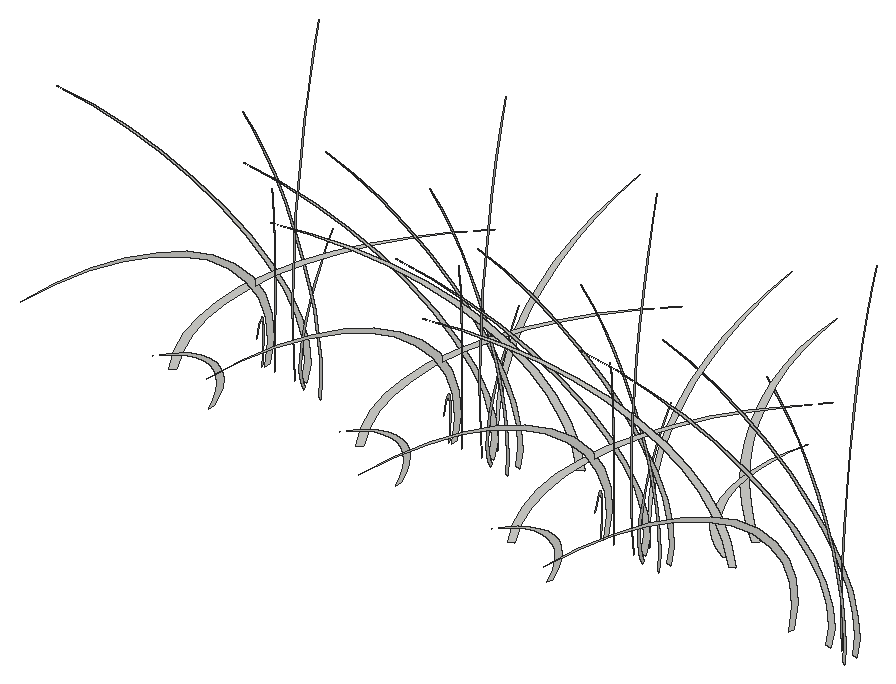
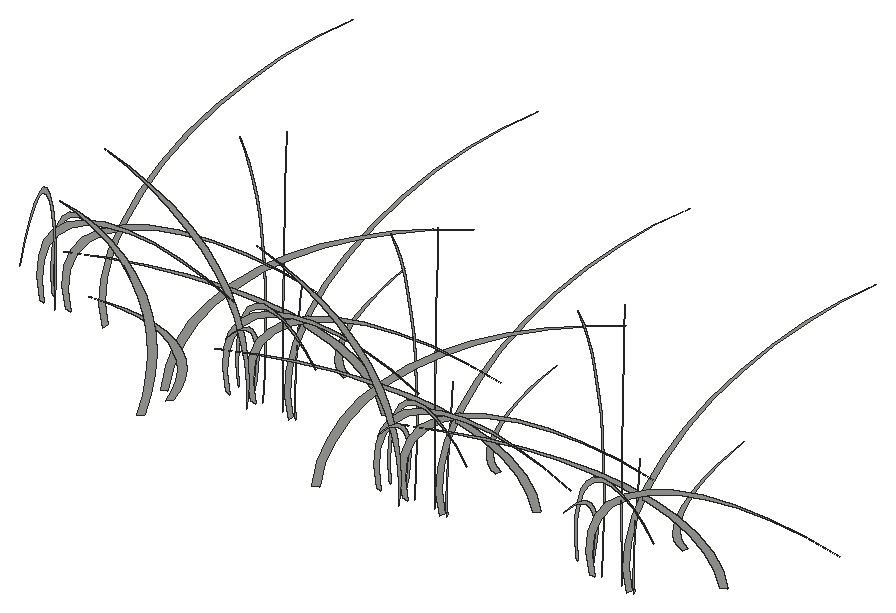
# SketchUp Ruby script. Lengths in inches.
U = 1.inch
M = Sketchup.active_model
def pt(a) = Geom::Point3d.new(a.map { |v| v * U })
def face(e, loops, mat)
  f = e.add_face(loops[0].map { |a| pt(a) })
  loops[1..].each { |l| e.add_face(l.map { |a| pt(a) }).erase! }
  f.material = f.back_material = mat if mat
  f
end
# faces: each face lists its corners as indices into pts; further lists are holes
def faces(e, pts, list, mat = nil) = list.each { |f| face(e, (f[0].is_a?(Array) ? f : [f]).map { |l| l.map { |i| pts[i] } }, mat) }
# xy, xz, yz: faces in a plane at the given z, y or x. An outline is a flat list of corners, or four numbers for a rectangle; further outlines are holes
def ring(l) = l.size == 4 ? [[l[0], l[1]], [l[2], l[1]], [l[2], l[3]], [l[0], l[3]]] : l.each_slice(2).to_a
def flat(e, list, mat, &to3) = list.each { |f| face(e, (f[0].is_a?(Array) ? f : [f]).map { |l| ring(l).map { |u, v| to3.(u, v) } }, mat) }
def xy(e, z, list, mat = nil) = flat(e, list, mat) { |x, y| [x, y, z] }
def xz(e, y, list, mat = nil) = flat(e, list, mat) { |x, z| [x, y, z] }
def yz(e, x, list, mat = nil) = flat(e, list, mat) { |y, z| [x, y, z] }
def lines(e, pts, list) = list.each { |a, b| e.add_line(pt(pts[a]), pt(pts[b])) }
# prism: a flat outline (further loops are holes) pulled along v
def prism(e, loops, v, mat = nil)
  f = face(e, loops, mat); d = Geom::Vector3d.new(v.map { |x| x * U })
  f.pushpull(f.normal.samedirection?(d) ? d.length : -d.length)
end
def box(e, o, s, mat = nil) = prism(e, [[o, [o[0] + s[0], o[1], o[2]], [o[0] + s[0], o[1] + s[1], o[2]], [o[0], o[1] + s[1], o[2]]]], [0, 0, s[2]], mat)
def at(x, y, z, deg = 0) = Geom::Transformation.translation(pt([x, y, z])) * Geom::Transformation.rotation(ORIGIN, Z_AXIS, deg.degrees)
def axes(o, x, y, z) = Geom::Transformation.new([*x, 0, *y, 0, *z, 0, *pt(o).to_a, 1])
def part(name) = M.definitions.add(name)
# library, detail: a bought-in or finely detailed component or shape, given as its bounding box
def library(name, o, s) = part(name).tap { |d| box(d.entities, o, s) }
def detail(e, o, s) = box(e.add_group.entities, o, s)
def put(e, d, t, mat = nil) = e.add_instance(d, t).tap { |i| i.material = mat if mat }
def group(e, t, mat = nil) = e.add_group.tap { |g| g.transformation = t; g.material = mat if mat }.entities
root = M.entities
g1 = group(root,at(438.46,264.24,0))
p = [[-0.1,-0.92,0],[-0.05,-0.41,0],[0,0,2.0625],[-0.02,-0.17,4.13],[-0.1,-0.9,6.16],[-0.24,-2.1875,8.1],
  [-0.44,-3.99,9.91],[-0.69,-6.27,11.52],[-0.99,-8.97,12.92],[-1.33,-12.02,14.05],[-1.69,-15.34,14.9],[-2.08,-18.86,15.45],
  [-2.48,-22.49,15.67],[-2.88,-26.13,15.5625],[-2.49,-22.56,15.58],[-2.1,-19.02,15.29],[-1.72,-15.6,14.71],[-1.37,-12.38,13.83],
  [-1.04,-9.43,12.68],[-0.75,-6.81,11.3],[-0.51,-4.6,9.7],[-0.3125,-2.84,7.9375],[-0.17,-1.5625,6.04],[-0.09,-0.81,4.05],
  [-0.07,-0.59,2.02]]
faces(g1,p,[[0,1,2,3,4,5,6,7,8,9,10,11,12,13,14,15,16,17,18,19,20,21,22,23,24]])
g2 = group(root,at(438.46,264.24,0))
p = [[-0.1,-0.92,0],[-0.05,-0.41,0],[0,0,2.0625],[-0.02,-0.17,4.13],[-0.1,-0.9,6.16],[-0.24,-2.1875,8.1],
  [-0.44,-3.99,9.91],[-0.69,-6.27,11.52],[-0.99,-8.97,12.92],[-1.33,-12.02,14.05],[-1.69,-15.34,14.9],[-2.08,-18.86,15.45],
  [-2.48,-22.49,15.67],[-2.88,-26.13,15.5625],[-2.49,-22.56,15.58],[-2.1,-19.02,15.29],[-1.72,-15.6,14.71],[-1.37,-12.38,13.83],
  [-1.04,-9.43,12.68],[-0.75,-6.81,11.3],[-0.51,-4.6,9.7],[-0.3125,-2.84,7.9375],[-0.17,-1.5625,6.04],[-0.09,-0.81,4.05],
  [-0.07,-0.59,2.02]]
faces(g2,p,[[0,1,2,3,4,5,6,7,8,9,10,11,12,13,14,15,16,17,18,19,20,21,22,23,24]])
g3 = group(root,at(419.3125,266.46,0))
p = [[-0.1,-0.92,0],[-0.05,-0.41,0],[0,0,2.0625],[-0.02,-0.17,4.13],[-0.1,-0.9,6.16],[-0.24,-2.1875,8.1],
  [-0.44,-3.99,9.91],[-0.69,-6.27,11.52],[-0.99,-8.97,12.92],[-1.33,-12.02,14.05],[-1.69,-15.34,14.9],[-2.08,-18.86,15.45],
  [-2.48,-22.49,15.67],[-2.88,-26.13,15.5625],[-2.49,-22.56,15.58],[-2.1,-19.02,15.29],[-1.72,-15.6,14.71],[-1.37,-12.38,13.83],
  [-1.04,-9.43,12.68],[-0.75,-6.81,11.3],[-0.51,-4.6,9.7],[-0.3125,-2.84,7.9375],[-0.17,-1.5625,6.04],[-0.09,-0.81,4.05],
  [-0.07,-0.59,2.02]]
faces(g3,p,[[0,1,2,3,4,5,6,7,8,9,10,11,12,13,14,15,16,17,18,19,20,21,22,23,24]])
g4 = group(root,at(419.3125,266.46,0))
p = [[-0.1,-0.92,0],[-0.05,-0.41,0],[0,0,2.0625],[-0.02,-0.17,4.13],[-0.1,-0.9,6.16],[-0.24,-2.1875,8.1],
  [-0.44,-3.99,9.91],[-0.69,-6.27,11.52],[-0.99,-8.97,12.92],[-1.33,-12.02,14.05],[-1.69,-15.34,14.9],[-2.08,-18.86,15.45],
  [-2.48,-22.49,15.67],[-2.88,-26.13,15.5625],[-2.49,-22.56,15.58],[-2.1,-19.02,15.29],[-1.72,-15.6,14.71],[-1.37,-12.38,13.83],
  [-1.04,-9.43,12.68],[-0.75,-6.81,11.3],[-0.51,-4.6,9.7],[-0.3125,-2.84,7.9375],[-0.17,-1.5625,6.04],[-0.09,-0.81,4.05],
  [-0.07,-0.59,2.02]]
faces(g4,p,[[0,1,2,3,4,5,6,7,8,9,10,11,12,13,14,15,16,17,18,19,20,21,22,23,24]])
g5 = group(root,at(420.11,259.55,0))
p = [[-0.91,-7.12,6.7],[-0.75,-5.82,6.27],[-0.6,-4.64,5.81],[-0.46,-3.6,5.31],[-0.35,-2.71,4.77],[-0.25,-1.97,4.21],
  [-0.18,-1.39,3.63],[-0.125,-0.98,3.03],[-0.09,-0.74,2.43],[-0.09,-0.67,1.8125],[-0.1,-0.77,1.2],[-0.13,-1.05,0.59],
  [-0.19,-1.49,0],[-0.12,-0.92,0],[-0.05,-0.42,0.6],[-0.01,-0.11,1.22],[0,0,1.84],[-0.01,-0.08,2.47],
  [-0.04,-0.35,3.09],[-0.1,-0.81,3.69],[-0.1875,-1.45,4.28],[-0.29,-2.27,4.84],[-0.42,-3.26,5.37],[-0.57,-4.41,5.86],
  [-0.73,-5.7,6.3]]
faces(g5,p,[[0,1,2,3,4,5,6,7,8,9,10,11,12,13,14,15,16,17,18,19,20,21,22,23,24]])
g6 = group(root,at(401.6,270.81,0))
p = [[-0.1,-0.92,0],[-0.05,-0.41,0],[0,0,2.0625],[-0.02,-0.17,4.13],[-0.1,-0.9,6.16],[-0.24,-2.1875,8.1],
  [-0.44,-3.99,9.91],[-0.69,-6.27,11.52],[-0.99,-8.97,12.92],[-1.33,-12.02,14.05],[-1.69,-15.34,14.9],[-2.08,-18.86,15.45],
  [-2.48,-22.49,15.67],[-2.88,-26.13,15.5625],[-2.49,-22.56,15.58],[-2.1,-19.02,15.29],[-1.72,-15.6,14.71],[-1.37,-12.38,13.83],
  [-1.04,-9.43,12.68],[-0.75,-6.81,11.3],[-0.51,-4.6,9.7],[-0.3125,-2.84,7.9375],[-0.17,-1.5625,6.04],[-0.09,-0.81,4.05],
  [-0.07,-0.59,2.02]]
faces(g6,p,[[0,1,2,3,4,5,6,7,8,9,10,11,12,13,14,15,16,17,18,19,20,21,22,23,24]])
g7 = group(root,at(401.6,270.81,0))
p = [[-0.1,-0.92,0],[-0.05,-0.41,0],[0,0,2.0625],[-0.02,-0.17,4.13],[-0.1,-0.9,6.16],[-0.24,-2.1875,8.1],
  [-0.44,-3.99,9.91],[-0.69,-6.27,11.52],[-0.99,-8.97,12.92],[-1.33,-12.02,14.05],[-1.69,-15.34,14.9],[-2.08,-18.86,15.45],
  [-2.48,-22.49,15.67],[-2.88,-26.13,15.5625],[-2.49,-22.56,15.58],[-2.1,-19.02,15.29],[-1.72,-15.6,14.71],[-1.37,-12.38,13.83],
  [-1.04,-9.43,12.68],[-0.75,-6.81,11.3],[-0.51,-4.6,9.7],[-0.3125,-2.84,7.9375],[-0.17,-1.5625,6.04],[-0.09,-0.81,4.05],
  [-0.07,-0.59,2.02]]
faces(g7,p,[[0,1,2,3,4,5,6,7,8,9,10,11,12,13,14,15,16,17,18,19,20,21,22,23,24]])
g8 = group(root,at(383.74,271.23,0))
p = [[-0.1,-0.92,0],[-0.05,-0.41,0],[0,0,2.0625],[-0.02,-0.17,4.13],[-0.1,-0.9,6.16],[-0.24,-2.1875,8.1],
  [-0.44,-3.99,9.91],[-0.69,-6.27,11.52],[-0.99,-8.97,12.92],[-1.33,-12.02,14.05],[-1.69,-15.34,14.9],[-2.08,-18.86,15.45],
  [-2.48,-22.49,15.67],[-2.88,-26.13,15.5625],[-2.49,-22.56,15.58],[-2.1,-19.02,15.29],[-1.72,-15.6,14.71],[-1.37,-12.38,13.83],
  [-1.04,-9.43,12.68],[-0.75,-6.81,11.3],[-0.51,-4.6,9.7],[-0.3125,-2.84,7.9375],[-0.17,-1.5625,6.04],[-0.09,-0.81,4.05],
  [-0.07,-0.59,2.02]]
faces(g8,p,[[0,1,2,3,4,5,6,7,8,9,10,11,12,13,14,15,16,17,18,19,20,21,22,23,24]])
g9 = group(root,at(383.74,271.23,0))
p = [[-0.1,-0.92,0],[-0.05,-0.41,0],[0,0,2.0625],[-0.02,-0.17,4.13],[-0.1,-0.9,6.16],[-0.24,-2.1875,8.1],
  [-0.44,-3.99,9.91],[-0.69,-6.27,11.52],[-0.99,-8.97,12.92],[-1.33,-12.02,14.05],[-1.69,-15.34,14.9],[-2.08,-18.86,15.45],
  [-2.48,-22.49,15.67],[-2.88,-26.13,15.5625],[-2.49,-22.56,15.58],[-2.1,-19.02,15.29],[-1.72,-15.6,14.71],[-1.37,-12.38,13.83],
  [-1.04,-9.43,12.68],[-0.75,-6.81,11.3],[-0.51,-4.6,9.7],[-0.3125,-2.84,7.9375],[-0.17,-1.5625,6.04],[-0.09,-0.81,4.05],
  [-0.07,-0.59,2.02]]
faces(g9,p,[[0,1,2,3,4,5,6,7,8,9,10,11,12,13,14,15,16,17,18,19,20,21,22,23,24]])
g10 = group(root,at(402.4,263.9,0))
p = [[-0.91,-7.12,6.7],[-0.75,-5.82,6.27],[-0.6,-4.64,5.81],[-0.46,-3.6,5.31],[-0.35,-2.71,4.77],[-0.25,-1.97,4.21],
  [-0.18,-1.39,3.63],[-0.125,-0.98,3.03],[-0.09,-0.74,2.43],[-0.09,-0.67,1.8125],[-0.1,-0.77,1.2],[-0.13,-1.05,0.59],
  [-0.19,-1.49,0],[-0.12,-0.92,0],[-0.05,-0.42,0.6],[-0.01,-0.11,1.22],[0,0,1.84],[-0.01,-0.08,2.47],
  [-0.04,-0.35,3.09],[-0.1,-0.81,3.69],[-0.1875,-1.45,4.28],[-0.29,-2.27,4.84],[-0.42,-3.26,5.37],[-0.57,-4.41,5.86],
  [-0.73,-5.7,6.3]]
faces(g10,p,[[0,1,2,3,4,5,6,7,8,9,10,11,12,13,14,15,16,17,18,19,20,21,22,23,24]])
g11 = group(root,at(384.54,264.32,0))
p = [[-0.91,-7.12,6.7],[-0.75,-5.82,6.27],[-0.6,-4.64,5.81],[-0.46,-3.6,5.31],[-0.35,-2.71,4.77],[-0.25,-1.97,4.21],
  [-0.18,-1.39,3.63],[-0.125,-0.98,3.03],[-0.09,-0.74,2.43],[-0.09,-0.67,1.8125],[-0.1,-0.77,1.2],[-0.13,-1.05,0.59],
  [-0.19,-1.49,0],[-0.12,-0.92,0],[-0.05,-0.42,0.6],[-0.01,-0.11,1.22],[0,0,1.84],[-0.01,-0.08,2.47],
  [-0.04,-0.35,3.09],[-0.1,-0.81,3.69],[-0.1875,-1.45,4.28],[-0.29,-2.27,4.84],[-0.42,-3.26,5.37],[-0.57,-4.41,5.86],
  [-0.73,-5.7,6.3]]
faces(g11,p,[[0,1,2,3,4,5,6,7,8,9,10,11,12,13,14,15,16,17,18,19,20,21,22,23,24]])
g12 = group(root,at(419.68,266.18,0))
p = [[0.57,-0.76,0],[0.25,-0.34,1.67],[0.0625,-0.09,3.36],[0,0,5.0625],[0.0625,-0.08,6.76],[0.25,-0.33,8.45],
  [0.5625,-0.75,10.12],[1,-1.34,11.77],[1.56,-2.08,13.4],[2.23,-2.99,14.98],[3.03,-4.05,16.53],[3.93,-5.26,18.02],
  [4.95,-6.62,19.46],[3.99,-5.34,18],[3.14,-4.2,16.49],[2.39,-3.19,14.9375],[1.74,-2.33,13.35],[1.2,-1.61,11.73],
  [0.77,-1.03,10.08],[0.46,-0.61,8.42],[0.25,-0.34,6.74],[0.16,-0.21,5.05],[0.18,-0.24,3.36],[0.32,-0.43,1.68]]
faces(g12,p,[[0,1,2,3,4,5,6,7,8,9,10,11,12,13,14,15,16,17,18,19,20,21,22,23]])
g13 = group(root,at(418.05,266.83,0))
p = [[5.52,-7.72,6.7],[4.47,-6.25,6.27],[3.52,-4.92,5.81],[2.68,-3.75,5.31],[1.96,-2.74,4.77],[1.37,-1.91,4.21],
  [0.9,-1.26,3.63],[0.57,-0.79,3.03],[0.37,-0.52,2.43],[0.31,-0.44,1.8125],[0.4,-0.56,1.2],[0.62,-0.87,0.59],
  [0.98,-1.37,0],[0.74,-1.03,0],[0.33,-0.46,0.59],[0.07,-0.1,1.19],[-0.04,0.05,1.81],[0.01,-0.02,2.43],
  [0.21,-0.3,3.04],[0.5625,-0.79,3.65],[1.0625,-1.49,4.23],[1.7,-2.38,4.8],[2.48,-3.47,5.33],[3.38,-4.73,5.83],
  [4.4,-6.15,6.29]]
faces(g13,p,[[0,1,2,3,4,5,6,7,8,9,10,11,12,13,14,15,16,17,18,19,20,21,22,23,24]])
g14 = group(root,at(429.37,268.4,0))
p = [[-19.18,-7.98,16.73],[-22.08,-9.1875,17.17],[-19.27,-8.02,16.64],[-16.57,-6.9,15.9],[-13.98,-5.82,14.96],[-11.56,-4.8125,13.84],
  [-9.32,-3.88,12.54],[-7.28,-3.03,11.08],[-5.47,-2.28,9.48],[-3.92,-1.63,7.76],[-2.63,-1.09,5.92],[-1.625,-0.68,4.01],
  [-0.91,-0.38,2.02],[-0.5,-0.21,0],[0,0,0],[-0.34,-0.14,2.07],[-1.01,-0.42,4.1],[-1.99,-0.83,6.07],
  [-3.29,-1.37,7.94],[-4.88,-2.03,9.7],[-6.74,-2.81,11.33],[-8.85,-3.68,12.79],[-11.18,-4.65,14.08],[-13.7,-5.7,15.17],
  [-16.375,-6.82,16.0625]]
faces(g14,p,[[0,1,2,3,4,5,6,7,8,9,10,11,12,13,14,15,16,17,18,19,20,21,22,23,24]])
g15 = group(root,at(442.7,263.3,0))
p = [[-0.98,0.17,0],[-0.43,0.08,0],[0,0,1.75],[-0.18,0.03,3.51],[-0.96,0.17,5.24],[-2.32,0.41,6.89],
  [-4.24,0.76,8.42],[-6.67,1.1875,9.8],[-9.54,1.7,10.98],[-12.78,2.28,11.95],[-16.32,2.91,12.67],[-20.06,3.57,13.13],
  [-23.91,4.26,13.32],[-27.78,4.95,13.23],[-23.98,4.27,13.25],[-20.22,3.6,13],[-16.59,2.96,12.5],[-13.16,2.34,11.75],
  [-10.02,1.79,10.78],[-7.25,1.29,9.6],[-4.89,0.87,8.25],[-3.02,0.54,6.75],[-1.66,0.3,5.13],[-0.86,0.15,3.44],
  [-0.63,0.11,1.72]]
faces(g15,p,[[0,1,2,3,4,5,6,7,8,9,10,11,12,13,14,15,16,17,18,19,20,21,22,23,24]])
g16 = group(root,at(442.7,263.3,0))
p = [[-0.98,0.17,0],[-0.43,0.08,0],[0,0,1.75],[-0.18,0.03,3.51],[-0.96,0.17,5.24],[-2.32,0.41,6.89],
  [-4.24,0.76,8.42],[-6.67,1.1875,9.8],[-9.54,1.7,10.98],[-12.78,2.28,11.95],[-16.32,2.91,12.67],[-20.06,3.57,13.13],
  [-23.91,4.26,13.32],[-27.78,4.95,13.23],[-23.98,4.27,13.25],[-20.22,3.6,13],[-16.59,2.96,12.5],[-13.16,2.34,11.75],
  [-10.02,1.79,10.78],[-7.25,1.29,9.6],[-4.89,0.87,8.25],[-3.02,0.54,6.75],[-1.66,0.3,5.13],[-0.86,0.15,3.44],
  [-0.63,0.11,1.72]]
faces(g16,p,[[0,1,2,3,4,5,6,7,8,9,10,11,12,13,14,15,16,17,18,19,20,21,22,23,24]])
g17 = group(root,at(401.97,270.53,0))
p = [[0.57,-0.76,0],[0.25,-0.34,1.67],[0.0625,-0.09,3.36],[0,0,5.0625],[0.0625,-0.08,6.76],[0.25,-0.33,8.45],
  [0.5625,-0.75,10.12],[1,-1.34,11.77],[1.56,-2.08,13.4],[2.23,-2.99,14.98],[3.03,-4.05,16.53],[3.93,-5.26,18.02],
  [4.95,-6.62,19.46],[3.99,-5.34,18],[3.14,-4.2,16.49],[2.39,-3.19,14.9375],[1.74,-2.33,13.35],[1.2,-1.61,11.73],
  [0.77,-1.03,10.08],[0.46,-0.61,8.42],[0.25,-0.34,6.74],[0.16,-0.21,5.05],[0.18,-0.24,3.36],[0.32,-0.43,1.68]]
faces(g17,p,[[0,1,2,3,4,5,6,7,8,9,10,11,12,13,14,15,16,17,18,19,20,21,22,23]])
g18 = group(root,at(400.35,271.18,0))
p = [[5.52,-7.72,6.7],[4.47,-6.25,6.27],[3.52,-4.92,5.81],[2.68,-3.75,5.31],[1.96,-2.74,4.77],[1.37,-1.91,4.21],
  [0.9,-1.26,3.63],[0.57,-0.79,3.03],[0.37,-0.52,2.43],[0.31,-0.44,1.8125],[0.4,-0.56,1.2],[0.62,-0.87,0.59],
  [0.98,-1.37,0],[0.74,-1.03,0],[0.33,-0.46,0.59],[0.07,-0.1,1.19],[-0.04,0.05,1.81],[0.01,-0.02,2.43],
  [0.21,-0.3,3.04],[0.5625,-0.79,3.65],[1.0625,-1.49,4.23],[1.7,-2.38,4.8],[2.48,-3.47,5.33],[3.38,-4.73,5.83],
  [4.4,-6.15,6.29]]
faces(g18,p,[[0,1,2,3,4,5,6,7,8,9,10,11,12,13,14,15,16,17,18,19,20,21,22,23,24]])
g19 = group(root,at(384.11,270.95,0))
p = [[0.57,-0.76,0],[0.25,-0.34,1.67],[0.0625,-0.09,3.36],[0,0,5.0625],[0.0625,-0.08,6.76],[0.25,-0.33,8.45],
  [0.5625,-0.75,10.12],[1,-1.34,11.77],[1.56,-2.08,13.4],[2.23,-2.99,14.98],[3.03,-4.05,16.53],[3.93,-5.26,18.02],
  [4.95,-6.62,19.46],[3.99,-5.34,18],[3.14,-4.2,16.49],[2.39,-3.19,14.9375],[1.74,-2.33,13.35],[1.2,-1.61,11.73],
  [0.77,-1.03,10.08],[0.46,-0.61,8.42],[0.25,-0.34,6.74],[0.16,-0.21,5.05],[0.18,-0.24,3.36],[0.32,-0.43,1.68]]
faces(g19,p,[[0,1,2,3,4,5,6,7,8,9,10,11,12,13,14,15,16,17,18,19,20,21,22,23]])
g20 = group(root,at(413.92,260.93,0))
p = [[17.17,11.7,12.375],[19.76,13.47,12.7],[17.25,11.76,12.31],[14.83,10.11,11.76],[12.52,8.53,11.07],[10.35,7.05,10.23],
  [8.34,5.68,9.27],[6.52,4.44,8.2],[4.9,3.34,7.01],[3.51,2.39,5.74],[2.35,1.6,4.38],[1.45,0.99,2.96],
  [0.82,0.56,1.5],[0.45,0.3,0],[0,0,0],[0.3,0.21,1.53],[0.9,0.61,3.03],[1.78,1.22,4.49],
  [2.95,2.01,5.875],[4.37,2.98,7.18],[6.03,4.11,8.375],[7.92,5.4,9.46],[10,6.82,10.41],[12.26,8.36,11.22],
  [14.66,9.99,11.88]]
faces(g20,p,[[0,1,2,3,4,5,6,7,8,9,10,11,12,13,14,15,16,17,18,19,20,21,22,23,24]])
g21 = group(root,at(382.48,271.6,0))
p = [[5.52,-7.72,6.7],[4.47,-6.25,6.27],[3.52,-4.92,5.81],[2.68,-3.75,5.31],[1.96,-2.74,4.77],[1.37,-1.91,4.21],
  [0.9,-1.26,3.63],[0.57,-0.79,3.03],[0.37,-0.52,2.43],[0.31,-0.44,1.8125],[0.4,-0.56,1.2],[0.62,-0.87,0.59],
  [0.98,-1.37,0],[0.74,-1.03,0],[0.33,-0.46,0.59],[0.07,-0.1,1.19],[-0.04,0.05,1.81],[0.01,-0.02,2.43],
  [0.21,-0.3,3.04],[0.5625,-0.79,3.65],[1.0625,-1.49,4.23],[1.7,-2.38,4.8],[2.48,-3.47,5.33],[3.38,-4.73,5.83],
  [4.4,-6.15,6.29]]
faces(g21,p,[[0,1,2,3,4,5,6,7,8,9,10,11,12,13,14,15,16,17,18,19,20,21,22,23,24]])
g22 = group(root,at(424.125,263.46,0))
p = [[-3.85,8.68,9.0625],[-3.11,7.03,8.49],[-2.45,5.54,7.85],[-1.87,4.22,7.18],[-1.37,3.08,6.45],[-0.95,2.15,5.7],
  [-0.625,1.41,4.91],[-0.39,0.89,4.1],[-0.26,0.58,3.28],[-0.22,0.49,2.45],[-0.28,0.625,1.625],[-0.43,0.97,0.8],
  [-0.68,1.54,0],[-0.52,1.16,0],[-0.23,0.52,0.8],[-0.05,0.11,1.61],[0.02,-0.06,2.45],[-0.01,0.02,3.28],
  [-0.15,0.33,4.11],[-0.39,0.89,4.93],[-0.74,1.67,5.72],[-1.1875,2.68,6.49],[-1.73,3.9,7.21],[-2.35,5.3125,7.88],
  [-3.0625,6.91,8.5]]
faces(g22,p,[[0,1,2,3,4,5,6,7,8,9,10,11,12,13,14,15,16,17,18,19,20,21,22,23,24]])
g23 = group(root,at(423.55,265.52,0))
p = [[-0.98,0.17,0],[-0.43,0.08,0],[0,0,1.75],[-0.18,0.03,3.51],[-0.96,0.17,5.24],[-2.32,0.41,6.89],
  [-4.24,0.76,8.42],[-6.67,1.1875,9.8],[-9.54,1.7,10.98],[-12.78,2.28,11.95],[-16.32,2.91,12.67],[-20.06,3.57,13.13],
  [-23.91,4.26,13.32],[-27.78,4.95,13.23],[-23.98,4.27,13.25],[-20.22,3.6,13],[-16.59,2.96,12.5],[-13.16,2.34,11.75],
  [-10.02,1.79,10.78],[-7.25,1.29,9.6],[-4.89,0.87,8.25],[-3.02,0.54,6.75],[-1.66,0.3,5.13],[-0.86,0.15,3.44],
  [-0.63,0.11,1.72]]
faces(g23,p,[[0,1,2,3,4,5,6,7,8,9,10,11,12,13,14,15,16,17,18,19,20,21,22,23,24]])
g24 = group(root,at(423.55,265.52,0))
p = [[-0.98,0.17,0],[-0.43,0.08,0],[0,0,1.75],[-0.18,0.03,3.51],[-0.96,0.17,5.24],[-2.32,0.41,6.89],
  [-4.24,0.76,8.42],[-6.67,1.1875,9.8],[-9.54,1.7,10.98],[-12.78,2.28,11.95],[-16.32,2.91,12.67],[-20.06,3.57,13.13],
  [-23.91,4.26,13.32],[-27.78,4.95,13.23],[-23.98,4.27,13.25],[-20.22,3.6,13],[-16.59,2.96,12.5],[-13.16,2.34,11.75],
  [-10.02,1.79,10.78],[-7.25,1.29,9.6],[-4.89,0.87,8.25],[-3.02,0.54,6.75],[-1.66,0.3,5.13],[-0.86,0.15,3.44],
  [-0.63,0.11,1.72]]
faces(g24,p,[[0,1,2,3,4,5,6,7,8,9,10,11,12,13,14,15,16,17,18,19,20,21,22,23,24]])
g25 = group(root,at(411.66,272.75,0))
p = [[-19.18,-7.98,16.73],[-22.08,-9.1875,17.17],[-19.27,-8.02,16.64],[-16.57,-6.9,15.9],[-13.98,-5.82,14.96],[-11.56,-4.8125,13.84],
  [-9.32,-3.88,12.54],[-7.28,-3.03,11.08],[-5.47,-2.28,9.48],[-3.92,-1.63,7.76],[-2.63,-1.09,5.92],[-1.625,-0.68,4.01],
  [-0.91,-0.38,2.02],[-0.5,-0.21,0],[0,0,0],[-0.34,-0.14,2.07],[-1.01,-0.42,4.1],[-1.99,-0.83,6.07],
  [-3.29,-1.37,7.94],[-4.88,-2.03,9.7],[-6.74,-2.81,11.33],[-8.85,-3.68,12.79],[-11.18,-4.65,14.08],[-13.7,-5.7,15.17],
  [-16.375,-6.82,16.0625]]
faces(g25,p,[[0,1,2,3,4,5,6,7,8,9,10,11,12,13,14,15,16,17,18,19,20,21,22,23,24]])
g26 = group(root,at(444.88,261.87,0))
p = [[-0.62,0.44,0],[-0.27,0.2,0],[0,0,1.68],[-0.11,0.08,3.37],[-0.6,0.43,5.03],[-1.46,1.05,6.61],
  [-2.67,1.92,8.08],[-4.2,3.02,9.4],[-6.01,4.32,10.54],[-8.05,5.79,11.47],[-10.28,7.39,12.16],[-12.64,9.08,12.61],
  [-15.07,10.83,12.79],[-17.5,12.58,12.7],[-15.11,10.86,12.72],[-12.74,9.16,12.48],[-10.45,7.51,12],[-8.29,5.96,11.29],
  [-6.32,4.54,10.35],[-4.57,3.28,9.22],[-3.08,2.21,7.92],[-1.9,1.37,6.48],[-1.05,0.75,4.93],[-0.54,0.39,3.31],
  [-0.4,0.29,1.65]]
faces(g26,p,[[0,1,2,3,4,5,6,7,8,9,10,11,12,13,14,15,16,17,18,19,20,21,22,23,24]])
g27 = group(root,at(422.66,264.42,0))
p = [[-0.4,0.86,0],[-0.18,0.38,2.26],[-0.05,0.1,4.55],[0,0,6.84],[-0.04,0.09,9.14],[-0.18,0.38,11.42],
  [-0.4,0.85,13.6875],[-0.71,1.51,15.92],[-1.1,2.36,18.12],[-1.58,3.38,20.26],[-2.14,4.58,22.35],[-2.79,5.95,24.37],
  [-3.51,7.48,26.3125],[-2.83,6.04,24.34],[-2.22,4.75,22.3],[-1.69,3.61,20.2],[-1.23,2.63,18.05],[-0.85,1.82,15.86],
  [-0.55,1.17,13.64],[-0.32,0.6875,11.38],[-0.18,0.38,9.11],[-0.11,0.24,6.83],[-0.13,0.28,4.54],[-0.23,0.48,2.27]]
faces(g27,p,[[0,1,2,3,4,5,6,7,8,9,10,11,12,13,14,15,16,17,18,19,20,21,22,23]])
g28 = group(root,at(445.05,263.26,0))
p = [[-0.93,0.35,0],[-0.41,0.16,0],[0,0,1.75],[-0.17,0.0625,3.51],[-0.91,0.34,5.24],[-2.21,0.83,6.89],
  [-4.03,1.52,8.42],[-6.34,2.39,9.8],[-9.0625,3.42,10.98],[-12.14,4.59,11.95],[-15.5,5.86,12.67],[-19.06,7.2,13.13],
  [-22.72,8.58,13.32],[-26.4,9.97,13.23],[-22.79,8.61,13.25],[-19.22,7.26,13],[-15.76,5.96,12.5],[-12.51,4.73,11.75],
  [-9.53,3.6,10.78],[-6.89,2.6,9.6],[-4.65,1.76,8.25],[-2.87,1.08,6.75],[-1.58,0.6,5.13],[-0.82,0.31,3.44],
  [-0.6,0.23,1.72]]
faces(g28,p,[[0,1,2,3,4,5,6,7,8,9,10,11,12,13,14,15,16,17,18,19,20,21,22,23,24]])
g29 = group(root,at(425.73,264.08,0))
p = [[-0.62,0.44,0],[-0.27,0.2,0],[0,0,1.68],[-0.11,0.08,3.37],[-0.6,0.43,5.03],[-1.46,1.05,6.61],
  [-2.67,1.92,8.08],[-4.2,3.02,9.4],[-6.01,4.32,10.54],[-8.05,5.79,11.47],[-10.28,7.39,12.16],[-12.64,9.08,12.61],
  [-15.07,10.83,12.79],[-17.5,12.58,12.7],[-15.11,10.86,12.72],[-12.74,9.16,12.48],[-10.45,7.51,12],[-8.29,5.96,11.29],
  [-6.32,4.54,10.35],[-4.57,3.28,9.22],[-3.08,2.21,7.92],[-1.9,1.37,6.48],[-1.05,0.75,4.93],[-0.54,0.39,3.31],
  [-0.4,0.29,1.65]]
faces(g29,p,[[0,1,2,3,4,5,6,7,8,9,10,11,12,13,14,15,16,17,18,19,20,21,22,23,24]])
g30 = group(root,at(422.47,266.66,0))
p = [[7.51,7.51,22.54],[6.3125,6.3125,20.88],[5.21,5.21,19.16],[4.21,4.21,17.39],[3.32,3.32,15.57],[2.52,2.52,13.71],
  [1.84,1.84,11.82],[1.27,1.27,9.89],[0.81,0.81,7.94],[0.46,0.46,5.97],[0.22,0.22,3.99],[0.1,0.1,2],
  [0.1,0.1,0],[0,0,2.01],[0.04,0.04,4.01],[0.21,0.21,6.01],[0.51,0.51,8],[0.95,0.95,9.97],
  [1.51,1.51,11.91],[2.21,2.21,13.81],[3.03,3.03,15.67],[3.98,3.98,17.48],[5.04,5.04,19.23],[6.22,6.22,20.92]]
faces(g30,p,[[0,1,2,3,4,5,6,7,8,9,10,11,12,13,14,15,16,17,18,19,20,21,22,23]])
g31 = group(root,at(425.9,265.48,0))
p = [[-0.93,0.35,0],[-0.41,0.16,0],[0,0,1.75],[-0.17,0.0625,3.51],[-0.91,0.34,5.24],[-2.21,0.83,6.89],
  [-4.03,1.52,8.42],[-6.34,2.39,9.8],[-9.0625,3.42,10.98],[-12.14,4.59,11.95],[-15.5,5.86,12.67],[-19.06,7.2,13.13],
  [-22.72,8.58,13.32],[-26.4,9.97,13.23],[-22.79,8.61,13.25],[-19.22,7.26,13],[-15.76,5.96,12.5],[-12.51,4.73,11.75],
  [-9.53,3.6,10.78],[-6.89,2.6,9.6],[-4.65,1.76,8.25],[-2.87,1.08,6.75],[-1.58,0.6,5.13],[-0.82,0.31,3.44],
  [-0.6,0.23,1.72]]
faces(g31,p,[[0,1,2,3,4,5,6,7,8,9,10,11,12,13,14,15,16,17,18,19,20,21,22,23,24]])
g32 = group(root,at(426.93,268.39,0))
p = [[5.08,5.08,9.0625],[4.15,4.15,8.49],[3.31,3.31,7.85],[2.57,2.57,7.18],[1.93,1.93,6.45],[1.41,1.41,5.7],
  [0.99,0.99,4.91],[0.7,0.7,4.1],[0.53,0.53,3.28],[0.48,0.48,2.45],[0.55,0.55,1.625],[0.75,0.75,0.8],
  [1.0625,1.0625,0],[0.65,0.65,0],[0.3,0.3,0.81],[0.08,0.08,1.65],[0,0,2.49],[0.06,0.06,3.34],
  [0.25,0.25,4.17],[0.58,0.58,4.99],[1.04,1.04,5.79],[1.62,1.62,6.54],[2.33,2.33,7.26],[3.14,3.14,7.92],
  [4.0625,4.0625,8.52]]
faces(g32,p,[[0,1,2,3,4,5,6,7,8,9,10,11,12,13,14,15,16,17,18,19,20,21,22,23,24]])
g33 = group(root,at(396.21,265.28,0))
p = [[17.17,11.7,12.375],[19.76,13.47,12.7],[17.25,11.76,12.31],[14.83,10.11,11.76],[12.52,8.53,11.07],[10.35,7.05,10.23],
  [8.34,5.68,9.27],[6.52,4.44,8.2],[4.9,3.34,7.01],[3.51,2.39,5.74],[2.35,1.6,4.38],[1.45,0.99,2.96],
  [0.82,0.56,1.5],[0.45,0.3,0],[0,0,0],[0.3,0.21,1.53],[0.9,0.61,3.03],[1.78,1.22,4.49],
  [2.95,2.01,5.875],[4.37,2.98,7.18],[6.03,4.11,8.375],[7.92,5.4,9.46],[10,6.82,10.41],[12.26,8.36,11.22],
  [14.66,9.99,11.88]]
faces(g33,p,[[0,1,2,3,4,5,6,7,8,9,10,11,12,13,14,15,16,17,18,19,20,21,22,23,24]])
g34 = group(root,at(406.41,267.81,0))
p = [[-3.85,8.68,9.0625],[-3.11,7.03,8.49],[-2.45,5.54,7.85],[-1.87,4.22,7.18],[-1.37,3.08,6.45],[-0.95,2.15,5.7],
  [-0.625,1.41,4.91],[-0.39,0.89,4.1],[-0.26,0.58,3.28],[-0.22,0.49,2.45],[-0.28,0.625,1.625],[-0.43,0.97,0.8],
  [-0.68,1.54,0],[-0.52,1.16,0],[-0.23,0.52,0.8],[-0.05,0.11,1.61],[0.02,-0.06,2.45],[-0.01,0.02,3.28],
  [-0.15,0.33,4.11],[-0.39,0.89,4.93],[-0.74,1.67,5.72],[-1.1875,2.68,6.49],[-1.73,3.9,7.21],[-2.35,5.3125,7.88],
  [-3.0625,6.91,8.5]]
faces(g34,p,[[0,1,2,3,4,5,6,7,8,9,10,11,12,13,14,15,16,17,18,19,20,21,22,23,24]])
g35 = group(root,at(405.84,269.87,0))
p = [[-0.98,0.17,0],[-0.43,0.08,0],[0,0,1.75],[-0.18,0.03,3.51],[-0.96,0.17,5.24],[-2.32,0.41,6.89],
  [-4.24,0.76,8.42],[-6.67,1.1875,9.8],[-9.54,1.7,10.98],[-12.78,2.28,11.95],[-16.32,2.91,12.67],[-20.06,3.57,13.13],
  [-23.91,4.26,13.32],[-27.78,4.95,13.23],[-23.98,4.27,13.25],[-20.22,3.6,13],[-16.59,2.96,12.5],[-13.16,2.34,11.75],
  [-10.02,1.79,10.78],[-7.25,1.29,9.6],[-4.89,0.87,8.25],[-3.02,0.54,6.75],[-1.66,0.3,5.13],[-0.86,0.15,3.44],
  [-0.63,0.11,1.72]]
faces(g35,p,[[0,1,2,3,4,5,6,7,8,9,10,11,12,13,14,15,16,17,18,19,20,21,22,23,24]])
g36 = group(root,at(405.84,269.87,0))
p = [[-0.98,0.17,0],[-0.43,0.08,0],[0,0,1.75],[-0.18,0.03,3.51],[-0.96,0.17,5.24],[-2.32,0.41,6.89],
  [-4.24,0.76,8.42],[-6.67,1.1875,9.8],[-9.54,1.7,10.98],[-12.78,2.28,11.95],[-16.32,2.91,12.67],[-20.06,3.57,13.13],
  [-23.91,4.26,13.32],[-27.78,4.95,13.23],[-23.98,4.27,13.25],[-20.22,3.6,13],[-16.59,2.96,12.5],[-13.16,2.34,11.75],
  [-10.02,1.79,10.78],[-7.25,1.29,9.6],[-4.89,0.87,8.25],[-3.02,0.54,6.75],[-1.66,0.3,5.13],[-0.86,0.15,3.44],
  [-0.63,0.11,1.72]]
faces(g36,p,[[0,1,2,3,4,5,6,7,8,9,10,11,12,13,14,15,16,17,18,19,20,21,22,23,24]])
g37 = group(root,at(378.35,265.69,0))
p = [[17.17,11.7,12.375],[19.76,13.47,12.7],[17.25,11.76,12.31],[14.83,10.11,11.76],[12.52,8.53,11.07],[10.35,7.05,10.23],
  [8.34,5.68,9.27],[6.52,4.44,8.2],[4.9,3.34,7.01],[3.51,2.39,5.74],[2.35,1.6,4.38],[1.45,0.99,2.96],
  [0.82,0.56,1.5],[0.45,0.3,0],[0,0,0],[0.3,0.21,1.53],[0.9,0.61,3.03],[1.78,1.22,4.49],
  [2.95,2.01,5.875],[4.37,2.98,7.18],[6.03,4.11,8.375],[7.92,5.4,9.46],[10,6.82,10.41],[12.26,8.36,11.22],
  [14.66,9.99,11.88]]
faces(g37,p,[[0,1,2,3,4,5,6,7,8,9,10,11,12,13,14,15,16,17,18,19,20,21,22,23,24]])
g38 = group(root,at(404.96,268.77,0))
p = [[-0.4,0.86,0],[-0.18,0.38,2.26],[-0.05,0.1,4.55],[0,0,6.84],[-0.04,0.09,9.14],[-0.18,0.38,11.42],
  [-0.4,0.85,13.6875],[-0.71,1.51,15.92],[-1.1,2.36,18.12],[-1.58,3.38,20.26],[-2.14,4.58,22.35],[-2.79,5.95,24.37],
  [-3.51,7.48,26.3125],[-2.83,6.04,24.34],[-2.22,4.75,22.3],[-1.69,3.61,20.2],[-1.23,2.63,18.05],[-0.85,1.82,15.86],
  [-0.55,1.17,13.64],[-0.32,0.6875,11.38],[-0.18,0.38,9.11],[-0.11,0.24,6.83],[-0.13,0.28,4.54],[-0.23,0.48,2.27]]
faces(g38,p,[[0,1,2,3,4,5,6,7,8,9,10,11,12,13,14,15,16,17,18,19,20,21,22,23]])
g39 = group(root,at(388.55,268.22,0))
p = [[-3.85,8.68,9.0625],[-3.11,7.03,8.49],[-2.45,5.54,7.85],[-1.87,4.22,7.18],[-1.37,3.08,6.45],[-0.95,2.15,5.7],
  [-0.625,1.41,4.91],[-0.39,0.89,4.1],[-0.26,0.58,3.28],[-0.22,0.49,2.45],[-0.28,0.625,1.625],[-0.43,0.97,0.8],
  [-0.68,1.54,0],[-0.52,1.16,0],[-0.23,0.52,0.8],[-0.05,0.11,1.61],[0.02,-0.06,2.45],[-0.01,0.02,3.28],
  [-0.15,0.33,4.11],[-0.39,0.89,4.93],[-0.74,1.67,5.72],[-1.1875,2.68,6.49],[-1.73,3.9,7.21],[-2.35,5.3125,7.88],
  [-3.0625,6.91,8.5]]
faces(g39,p,[[0,1,2,3,4,5,6,7,8,9,10,11,12,13,14,15,16,17,18,19,20,21,22,23,24]])
g40 = group(root,at(387.98,270.28,0))
p = [[-0.98,0.17,0],[-0.43,0.08,0],[0,0,1.75],[-0.18,0.03,3.51],[-0.96,0.17,5.24],[-2.32,0.41,6.89],
  [-4.24,0.76,8.42],[-6.67,1.1875,9.8],[-9.54,1.7,10.98],[-12.78,2.28,11.95],[-16.32,2.91,12.67],[-20.06,3.57,13.13],
  [-23.91,4.26,13.32],[-27.78,4.95,13.23],[-23.98,4.27,13.25],[-20.22,3.6,13],[-16.59,2.96,12.5],[-13.16,2.34,11.75],
  [-10.02,1.79,10.78],[-7.25,1.29,9.6],[-4.89,0.87,8.25],[-3.02,0.54,6.75],[-1.66,0.3,5.13],[-0.86,0.15,3.44],
  [-0.63,0.11,1.72]]
faces(g40,p,[[0,1,2,3,4,5,6,7,8,9,10,11,12,13,14,15,16,17,18,19,20,21,22,23,24]])
g41 = group(root,at(387.98,270.28,0))
p = [[-0.98,0.17,0],[-0.43,0.08,0],[0,0,1.75],[-0.18,0.03,3.51],[-0.96,0.17,5.24],[-2.32,0.41,6.89],
  [-4.24,0.76,8.42],[-6.67,1.1875,9.8],[-9.54,1.7,10.98],[-12.78,2.28,11.95],[-16.32,2.91,12.67],[-20.06,3.57,13.13],
  [-23.91,4.26,13.32],[-27.78,4.95,13.23],[-23.98,4.27,13.25],[-20.22,3.6,13],[-16.59,2.96,12.5],[-13.16,2.34,11.75],
  [-10.02,1.79,10.78],[-7.25,1.29,9.6],[-4.89,0.87,8.25],[-3.02,0.54,6.75],[-1.66,0.3,5.13],[-0.86,0.15,3.44],
  [-0.63,0.11,1.72]]
faces(g41,p,[[0,1,2,3,4,5,6,7,8,9,10,11,12,13,14,15,16,17,18,19,20,21,22,23,24]])
g42 = group(root,at(387.09,269.1875,0))
p = [[-0.4,0.86,0],[-0.18,0.38,2.26],[-0.05,0.1,4.55],[0,0,6.84],[-0.04,0.09,9.14],[-0.18,0.38,11.42],
  [-0.4,0.85,13.6875],[-0.71,1.51,15.92],[-1.1,2.36,18.12],[-1.58,3.38,20.26],[-2.14,4.58,22.35],[-2.79,5.95,24.37],
  [-3.51,7.48,26.3125],[-2.83,6.04,24.34],[-2.22,4.75,22.3],[-1.69,3.61,20.2],[-1.23,2.63,18.05],[-0.85,1.82,15.86],
  [-0.55,1.17,13.64],[-0.32,0.6875,11.38],[-0.18,0.38,9.11],[-0.11,0.24,6.83],[-0.13,0.28,4.54],[-0.23,0.48,2.27]]
faces(g42,p,[[0,1,2,3,4,5,6,7,8,9,10,11,12,13,14,15,16,17,18,19,20,21,22,23]])
g43 = group(root,at(427.27,271.47,0))
p = [[5.08,5.08,18.42],[4.15,4.15,17.25],[3.31,3.31,15.97],[2.57,2.57,14.59],[1.93,1.93,13.12],[1.41,1.41,11.58],
  [0.99,0.99,9.98],[0.7,0.7,8.34],[0.53,0.53,6.67],[0.48,0.48,4.99],[0.55,0.55,3.3],[0.75,0.75,1.63],
  [1.0625,1.0625,0],[0.65,0.65,0],[0.3,0.3,1.66],[0.08,0.08,3.35],[0,0,5.07],[0.06,0.06,6.79],
  [0.25,0.25,8.49],[0.58,0.58,10.15],[1.04,1.04,11.76],[1.62,1.62,13.3],[2.33,2.33,14.75],[3.14,3.14,16.1],
  [4.0625,4.0625,17.33]]
faces(g43,p,[[0,1,2,3,4,5,6,7,8,9,10,11,12,13,14,15,16,17,18,19,20,21,22,23,24]])
g44 = group(root,at(443.41,263.15,0))
p = [[-0.5,0.78,0],[-0.22,0.34,0],[0,0,2.37],[-0.09,0.14,4.75],[-0.49,0.76,7.08],[-1.2,1.84,9.32],
  [-2.1875,3.37,11.39],[-3.4375,5.29,13.25],[-4.92,7.57,14.85],[-6.59,10.14,16.15],[-8.41,12.95,17.13],[-10.34,15.92,17.75],
  [-12.32,18.97,18.01],[-14.32,22.05,17.89],[-12.36,19.03,17.91],[-10.42,16.05,17.58],[-8.55,13.16,16.9],[-6.78,10.45,15.89],
  [-5.17,7.96,14.58],[-3.73,5.75,12.99],[-2.52,3.88,11.15],[-1.55,2.39,9.125],[-0.86,1.32,6.94],[-0.44,0.68,4.66],
  [-0.33,0.5,2.33]]
faces(g44,p,[[0,1,2,3,4,5,6,7,8,9,10,11,12,13,14,15,16,17,18,19,20,21,22,23,24]])
g45 = group(root,at(408.02,268.43,0))
p = [[-0.62,0.44,0],[-0.27,0.2,0],[0,0,1.68],[-0.11,0.08,3.37],[-0.6,0.43,5.03],[-1.46,1.05,6.61],
  [-2.67,1.92,8.08],[-4.2,3.02,9.4],[-6.01,4.32,10.54],[-8.05,5.79,11.47],[-10.28,7.39,12.16],[-12.64,9.08,12.61],
  [-15.07,10.83,12.79],[-17.5,12.58,12.7],[-15.11,10.86,12.72],[-12.74,9.16,12.48],[-10.45,7.51,12],[-8.29,5.96,11.29],
  [-6.32,4.54,10.35],[-4.57,3.28,9.22],[-3.08,2.21,7.92],[-1.9,1.37,6.48],[-1.05,0.75,4.93],[-0.54,0.39,3.31],
  [-0.4,0.29,1.65]]
faces(g45,p,[[0,1,2,3,4,5,6,7,8,9,10,11,12,13,14,15,16,17,18,19,20,21,22,23,24]])
g46 = group(root,at(404.76,271.01,0))
p = [[7.51,7.51,22.54],[6.3125,6.3125,20.88],[5.21,5.21,19.16],[4.21,4.21,17.39],[3.32,3.32,15.57],[2.52,2.52,13.71],
  [1.84,1.84,11.82],[1.27,1.27,9.89],[0.81,0.81,7.94],[0.46,0.46,5.97],[0.22,0.22,3.99],[0.1,0.1,2],
  [0.1,0.1,0],[0,0,2.01],[0.04,0.04,4.01],[0.21,0.21,6.01],[0.51,0.51,8],[0.95,0.95,9.97],
  [1.51,1.51,11.91],[2.21,2.21,13.81],[3.03,3.03,15.67],[3.98,3.98,17.48],[5.04,5.04,19.23],[6.22,6.22,20.92]]
faces(g46,p,[[0,1,2,3,4,5,6,7,8,9,10,11,12,13,14,15,16,17,18,19,20,21,22,23]])
g47 = group(root,at(408.1875,269.83,0))
p = [[-0.93,0.35,0],[-0.41,0.16,0],[0,0,1.75],[-0.17,0.0625,3.51],[-0.91,0.34,5.24],[-2.21,0.83,6.89],
  [-4.03,1.52,8.42],[-6.34,2.39,9.8],[-9.0625,3.42,10.98],[-12.14,4.59,11.95],[-15.5,5.86,12.67],[-19.06,7.2,13.13],
  [-22.72,8.58,13.32],[-26.4,9.97,13.23],[-22.79,8.61,13.25],[-19.22,7.26,13],[-15.76,5.96,12.5],[-12.51,4.73,11.75],
  [-9.53,3.6,10.78],[-6.89,2.6,9.6],[-4.65,1.76,8.25],[-2.87,1.08,6.75],[-1.58,0.6,5.13],[-0.82,0.31,3.44],
  [-0.6,0.23,1.72]]
faces(g47,p,[[0,1,2,3,4,5,6,7,8,9,10,11,12,13,14,15,16,17,18,19,20,21,22,23,24]])
g48 = group(root,at(390.16,268.85,0))
p = [[-0.62,0.44,0],[-0.27,0.2,0],[0,0,1.68],[-0.11,0.08,3.37],[-0.6,0.43,5.03],[-1.46,1.05,6.61],
  [-2.67,1.92,8.08],[-4.2,3.02,9.4],[-6.01,4.32,10.54],[-8.05,5.79,11.47],[-10.28,7.39,12.16],[-12.64,9.08,12.61],
  [-15.07,10.83,12.79],[-17.5,12.58,12.7],[-15.11,10.86,12.72],[-12.74,9.16,12.48],[-10.45,7.51,12],[-8.29,5.96,11.29],
  [-6.32,4.54,10.35],[-4.57,3.28,9.22],[-3.08,2.21,7.92],[-1.9,1.37,6.48],[-1.05,0.75,4.93],[-0.54,0.39,3.31],
  [-0.4,0.29,1.65]]
faces(g48,p,[[0,1,2,3,4,5,6,7,8,9,10,11,12,13,14,15,16,17,18,19,20,21,22,23,24]])
